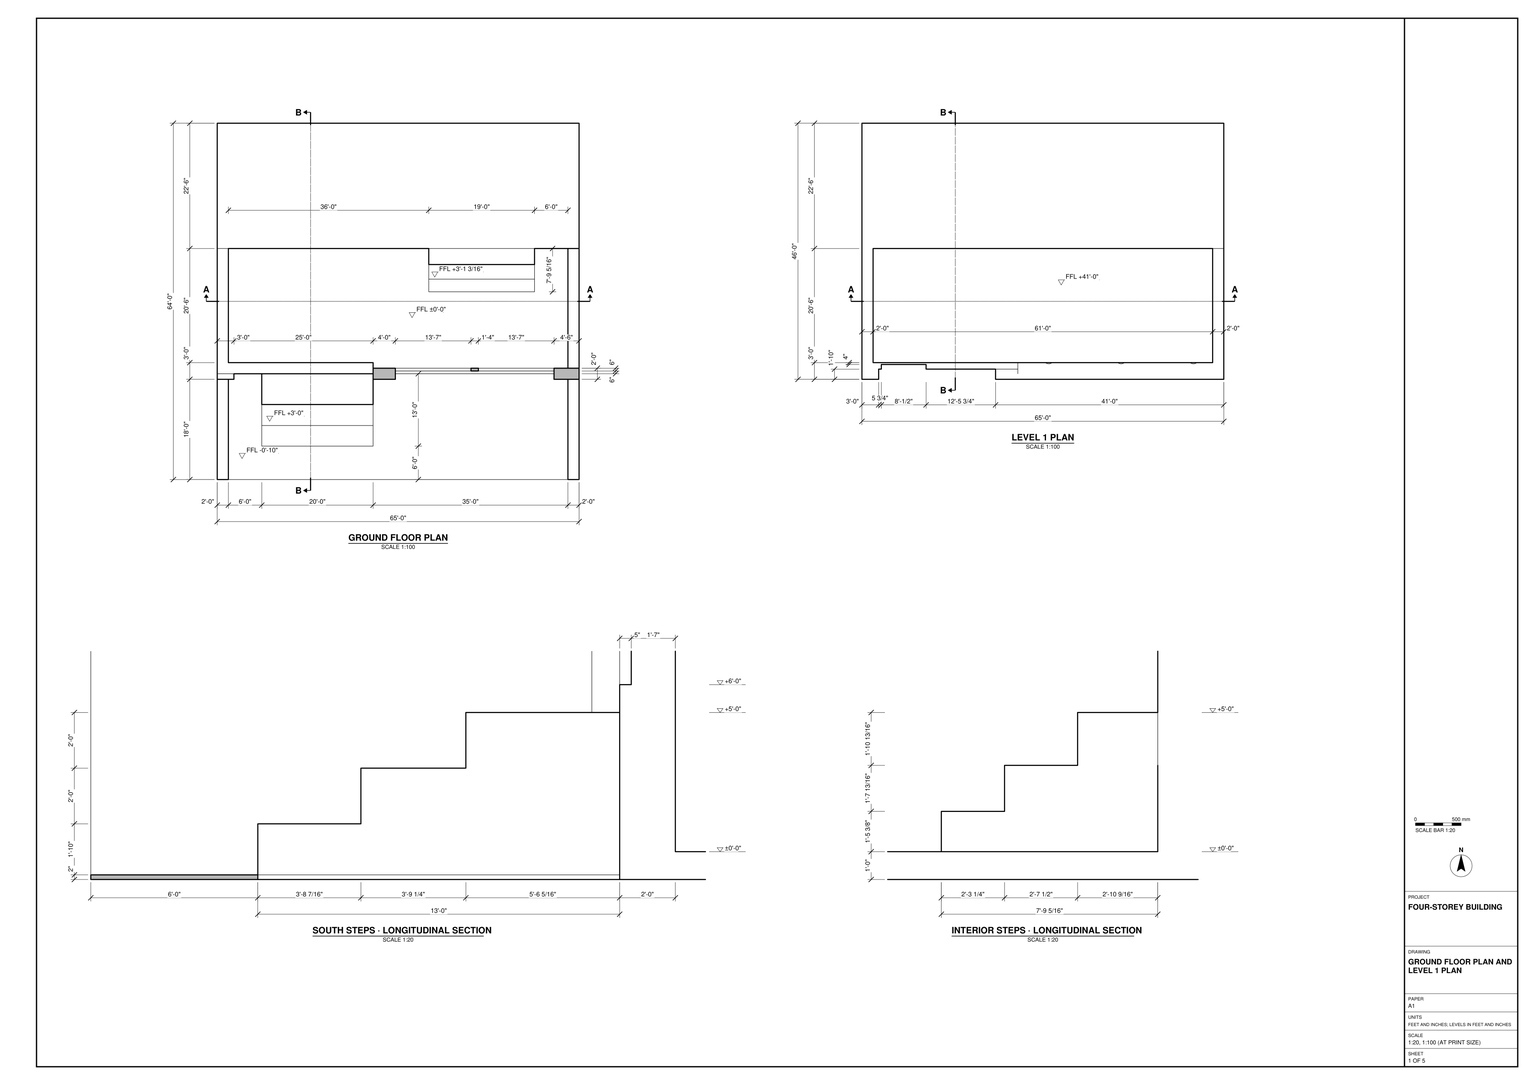
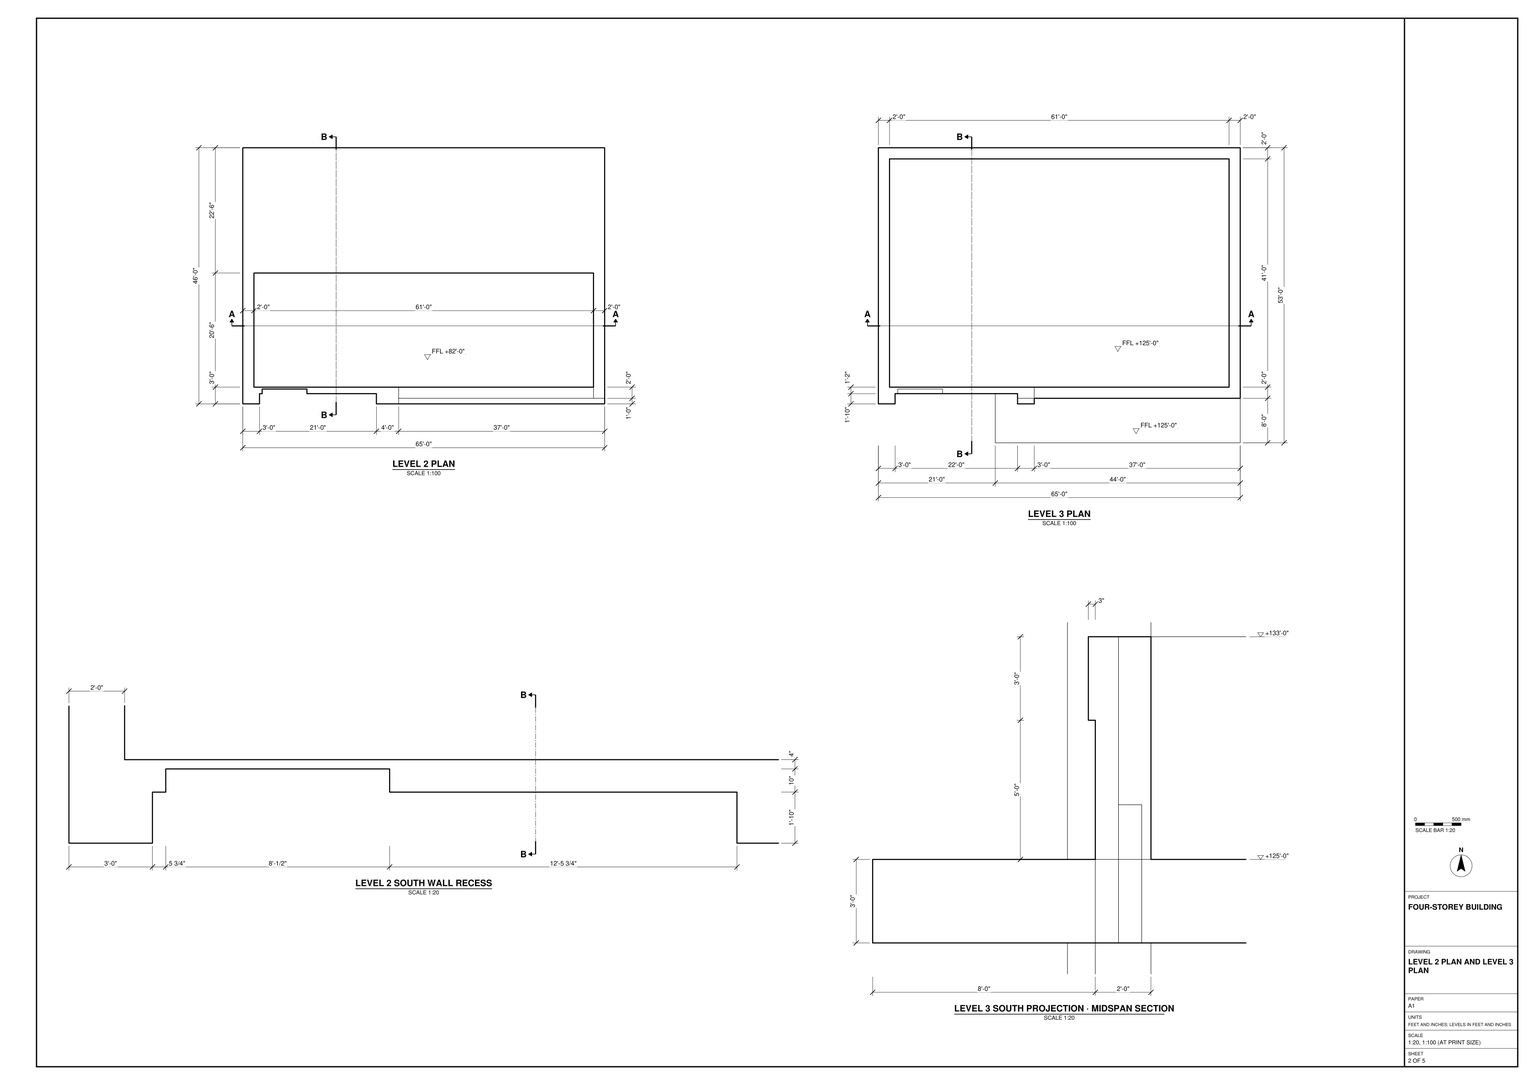
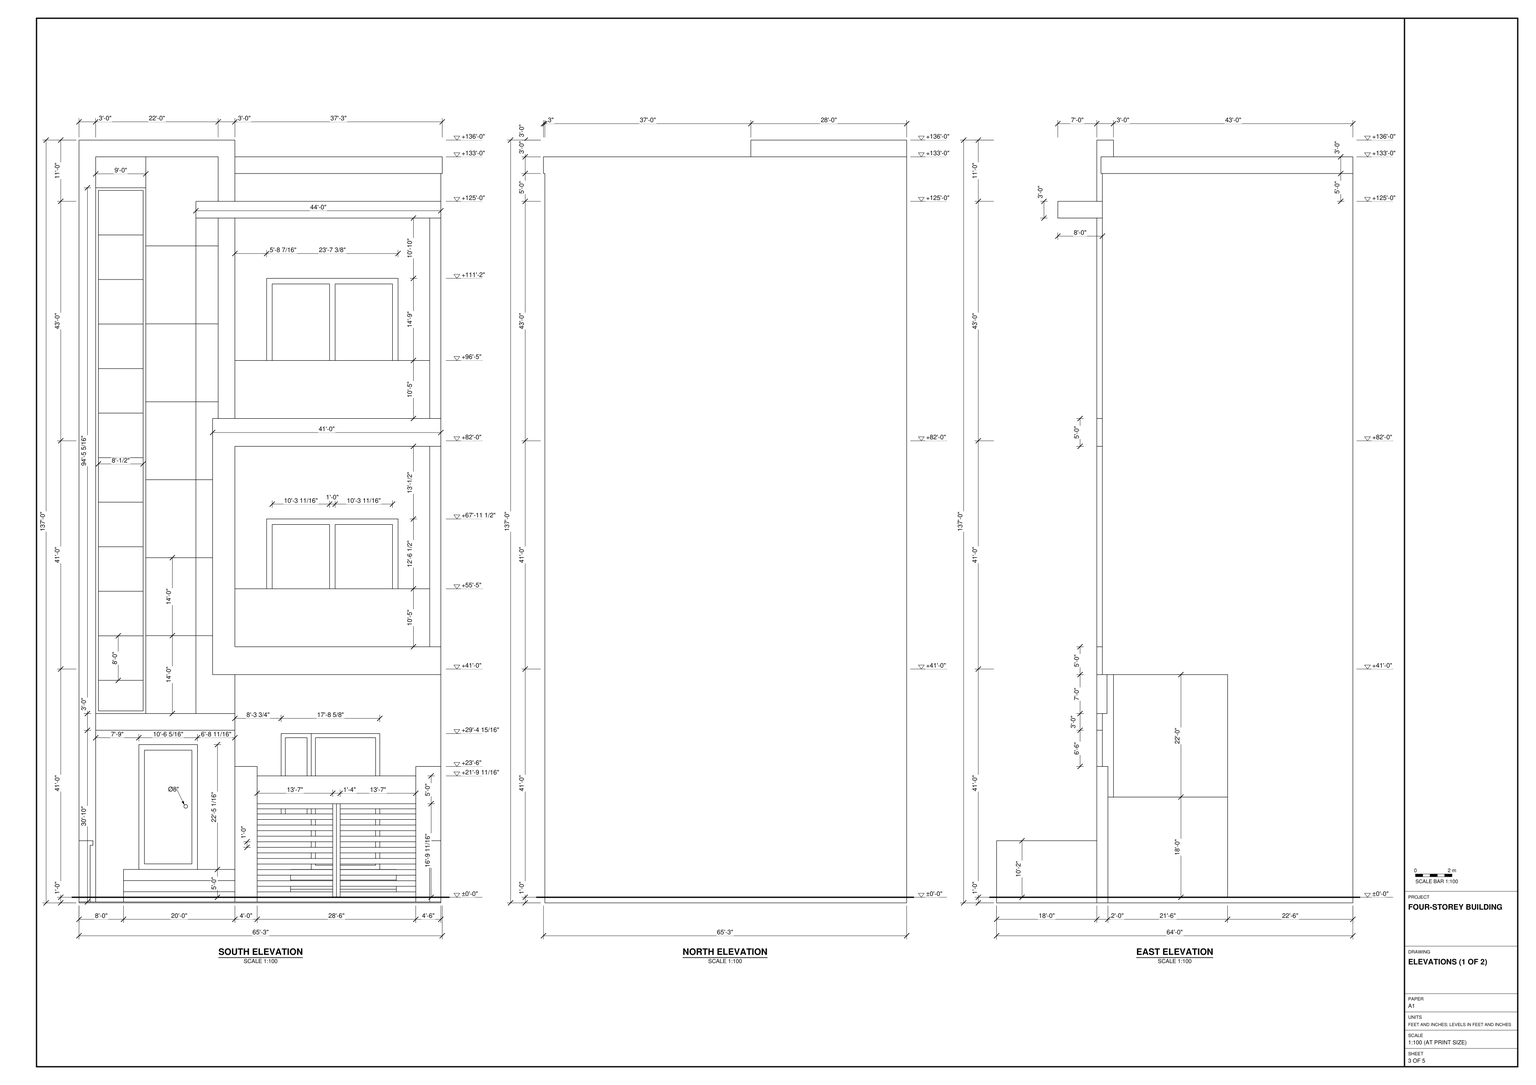
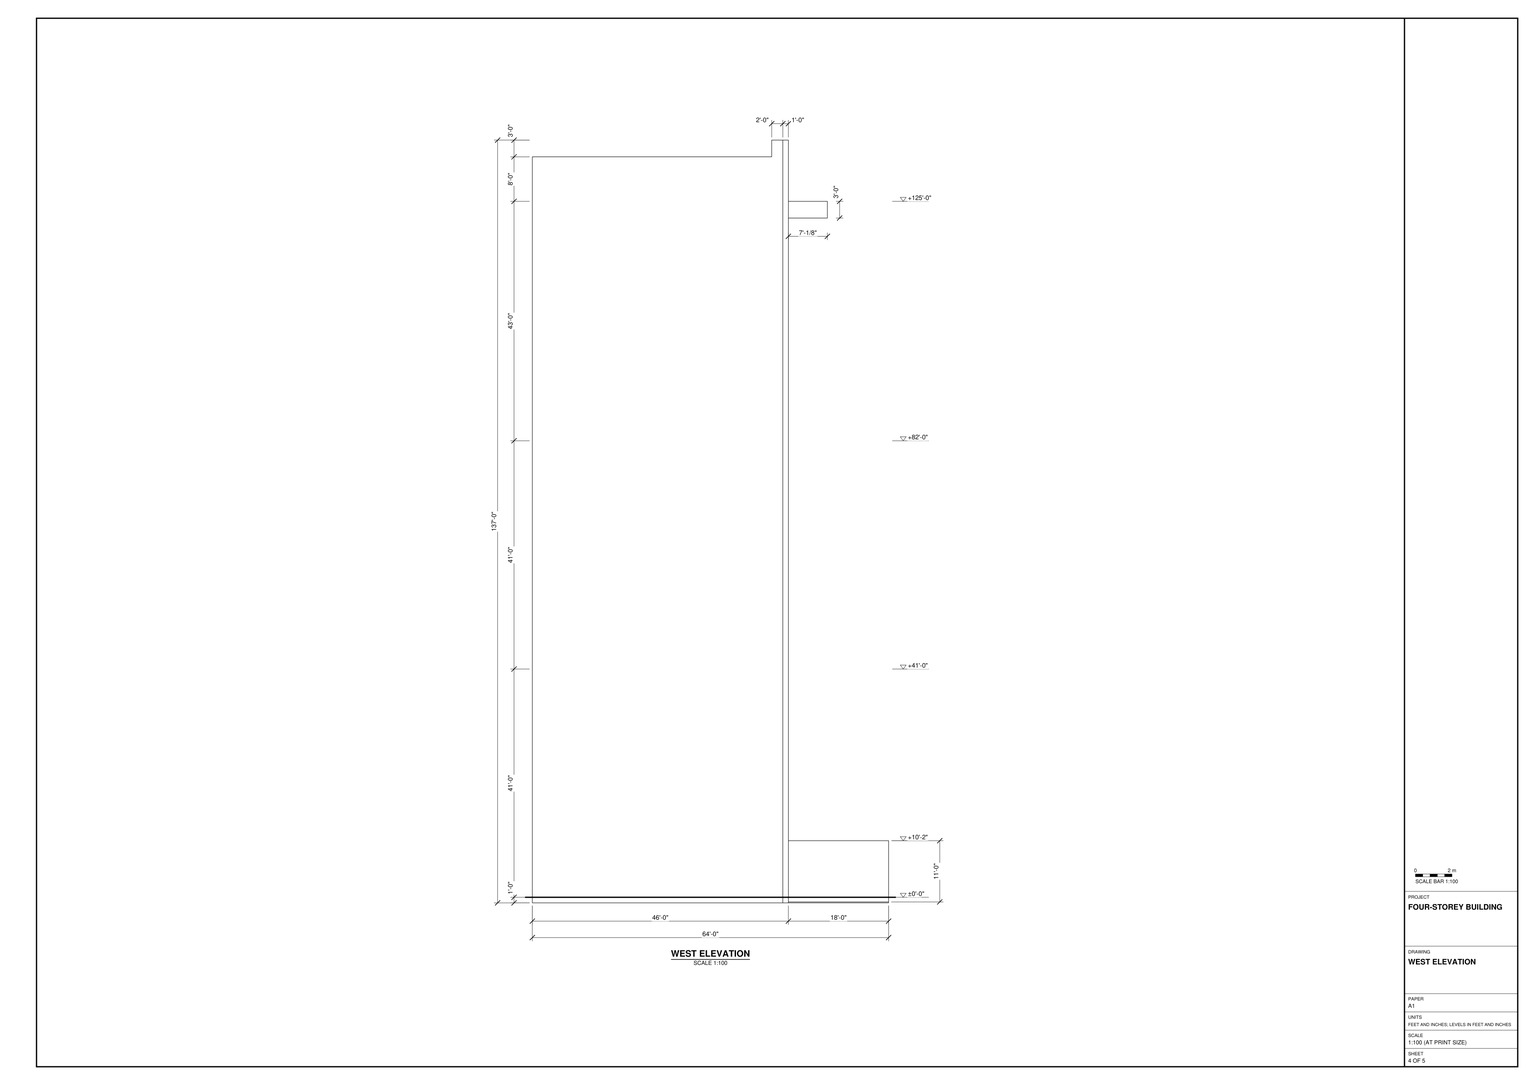
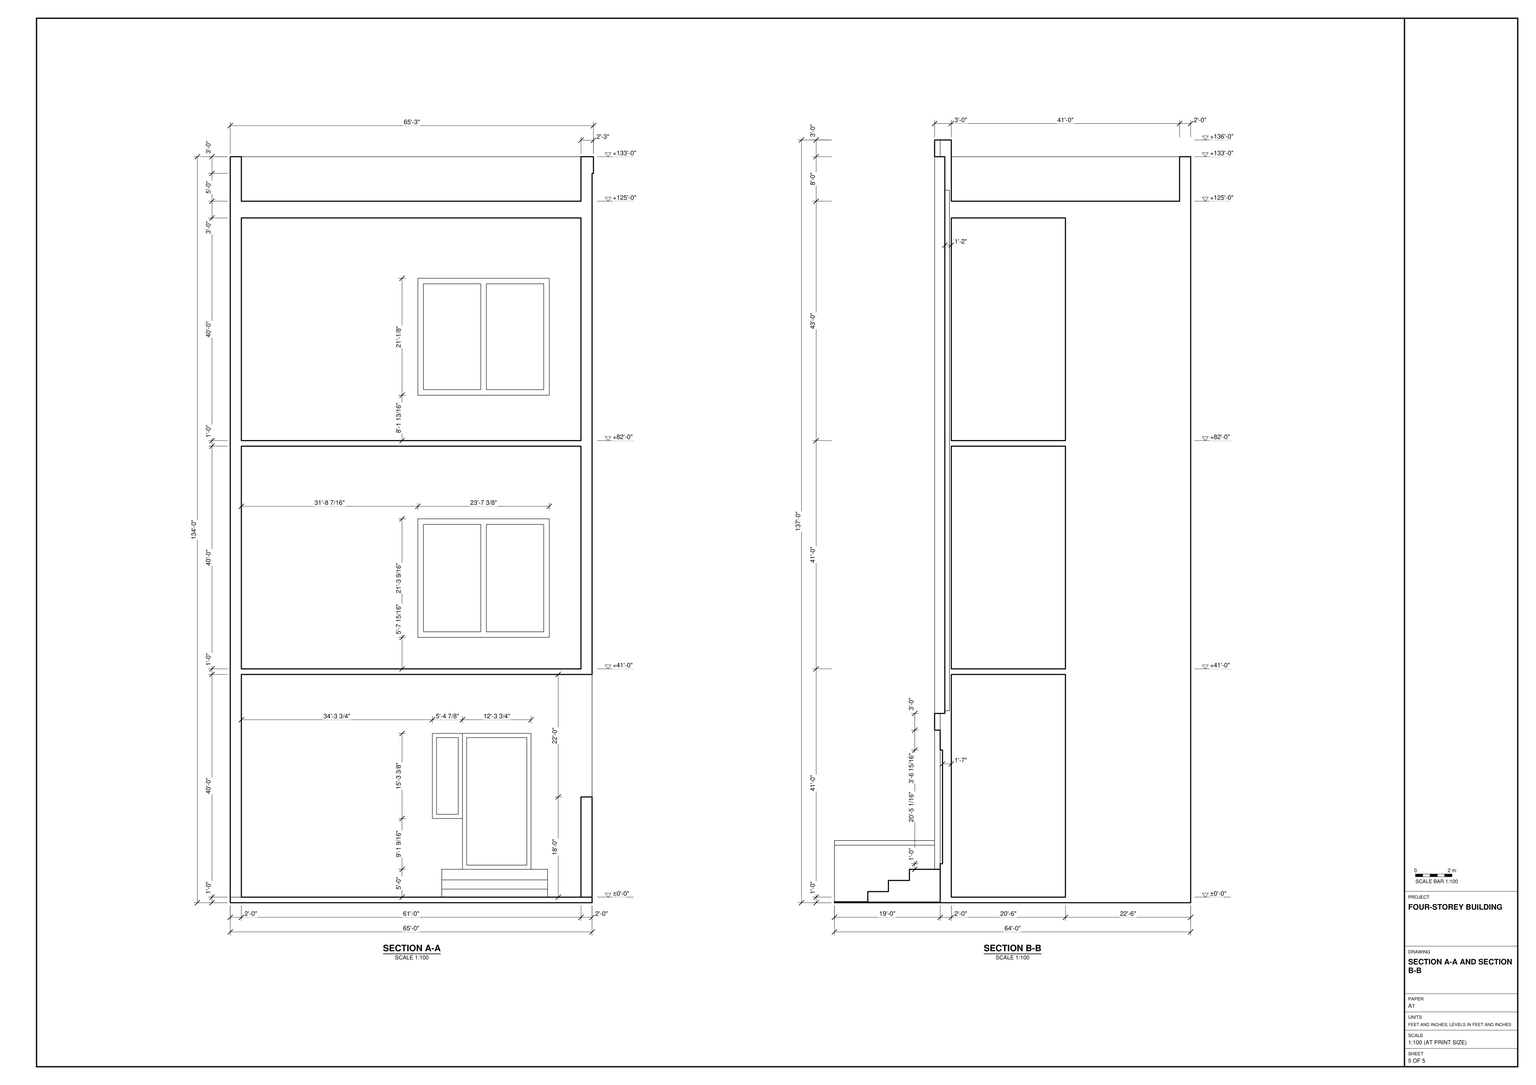
Build the four-storey building in SketchUp from task_files/diagram_01.pdf. Work in feet and inches. Set out the model with an overall east–west width of 65'-3", a north–south depth of 64'-0" and a total height of 137'-0". Use finished floor levels of ±0'-0", +41'-0", +82'-0" and +125'-0".

Follow the plans for the wall thicknesses, slab outlines and setbacks at each level. At ground level, extend the side walls along the south forecourt. Model the broad steps up to the entrance and the separate interior steps using their respective longitudinal sections. Place the entrance door to the left of the horizontal-slat gate as seen in the south elevation.

Build the tall, narrow panelled bay above the entrance and the paired upper-floor openings to its right. Give the facade its drawn depth: form the projecting surrounds, the level 2 wall recess and the level 3 slab projection rather than drawing their outlines on a flat wall. Finish the roof with the stepped parapet profile shown in elevation.

Keep walls, slabs and roof elements in separate groups or components, do the same for each furniture or joinery piece shown, and use components for repeated parts. Any decor or loose items shown may be suitable library components. Save one SketchUp model as output_files/four_storey_building_with_its_stepped_south_facade.skp.

# SketchUp Ruby script. Lengths in inches.
U = 1.inch
M = Sketchup.active_model
def pt(a) = Geom::Point3d.new(a.map { |v| v * U })
def face(e, loops, mat)
  f = e.add_face(loops[0].map { |a| pt(a) })
  loops[1..].each { |l| e.add_face(l.map { |a| pt(a) }).erase! }
  f.material = f.back_material = mat if mat
  f
end
# faces: each face lists its corners as indices into pts; further lists are holes
def faces(e, pts, list, mat = nil) = list.each { |f| face(e, (f[0].is_a?(Array) ? f : [f]).map { |l| l.map { |i| pts[i] } }, mat) }
# xy, xz, yz: faces in a plane at the given z, y or x. An outline is a flat list of corners, or four numbers for a rectangle; further outlines are holes
def ring(l) = l.size == 4 ? [[l[0], l[1]], [l[2], l[1]], [l[2], l[3]], [l[0], l[3]]] : l.each_slice(2).to_a
def flat(e, list, mat, &to3) = list.each { |f| face(e, (f[0].is_a?(Array) ? f : [f]).map { |l| ring(l).map { |u, v| to3.(u, v) } }, mat) }
def xy(e, z, list, mat = nil) = flat(e, list, mat) { |x, y| [x, y, z] }
def xz(e, y, list, mat = nil) = flat(e, list, mat) { |x, z| [x, y, z] }
def yz(e, x, list, mat = nil) = flat(e, list, mat) { |y, z| [x, y, z] }
def lines(e, pts, list) = list.each { |a, b| e.add_line(pt(pts[a]), pt(pts[b])) }
# prism: a flat outline (further loops are holes) pulled along v
def prism(e, loops, v, mat = nil)
  f = face(e, loops, mat); d = Geom::Vector3d.new(v.map { |x| x * U })
  f.pushpull(f.normal.samedirection?(d) ? d.length : -d.length)
end
def box(e, o, s, mat = nil) = prism(e, [[o, [o[0] + s[0], o[1], o[2]], [o[0] + s[0], o[1] + s[1], o[2]], [o[0], o[1] + s[1], o[2]]]], [0, 0, s[2]], mat)
def at(x, y, z, deg = 0) = Geom::Transformation.translation(pt([x, y, z])) * Geom::Transformation.rotation(ORIGIN, Z_AXIS, deg.degrees)
def axes(o, x, y, z) = Geom::Transformation.new([*x, 0, *y, 0, *z, 0, *pt(o).to_a, 1])
def part(name) = M.definitions.add(name)
# library, detail: a bought-in or finely detailed component or shape, given as its bounding box
def library(name, o, s) = part(name).tap { |d| box(d.entities, o, s) }
def detail(e, o, s) = box(e.add_group.entities, o, s)
def put(e, d, t, mat = nil) = e.add_instance(d, t).tap { |i| i.material = mat if mat }
def group(e, t, mat = nil) = e.add_group.tap { |g| g.transformation = t; g.material = mat if mat }.entities
root = M.entities
M.materials.add("[0035_Tan]").color = [178, 153, 119]
M.materials.add("[0111_SlateGray]").color = [41, 47, 53]
M.materials.add("[0135_DarkGray]").color = [81, 81, 81]
M.materials.add("[0137_Black]").color = [0, 0, 0]
M.materials.add("[Cladding Stucco White]").color = [173, 173, 173]
M.materials.add("[Granite Dark Gray]").color = [79, 77, 77]
M.materials.add("[Grass Dark Green]").color = [106, 157, 55]
M.materials.add("[Pavers Driveway Brick]").color = [176, 130, 106]
M.materials.add("[Pavers Flagstone Gray]").color = [162, 162, 162]
M.materials.add("[Stone Masonry Multi]").color = [226, 218, 204]
M.materials.add("[Stone Vein Gray]").color = [166, 165, 165]
M.materials.add("[Translucent Glass Blue]").color = [45, 67, 107]
M.materials["[Translucent Glass Blue]"].alpha = 0.5
M.materials.add("[Translucent Glass Gray]").color = [211, 211, 211]
M.materials["[Translucent Glass Gray]"].alpha = 0.5
M.materials.add("[Translucent Glass Gray]1").color = [128, 128, 128]
M.materials["[Translucent Glass Gray]1"].alpha = 0.5
M.materials.add("[Wood Bamboo]").color = [177, 105, 43]
M.materials.add("[Wood Veneer 01]").color = [120, 70, 37]
xy(root,0,[[0,0,0,216,36,216,36,228,96,228,96,72,336,72,336,216,384,216,384,228,726,228,726,216,780,216,780,0],[96,72,336,228],[0,216,36,228],[336,216,384,228],[726,216,780,228],
  [0,228,780,768]])
xy(root,2,[[0,0,24,216]])
xy(root,2,[[24,0,756,0,756,216,726,216,726,228,384,228,384,216,336,216,336,72,96,72,96,228,36,228,36,216,24,216]],"[Pavers Driveway Brick]")
xy(root,12,[[384,234,726,240],[756,240,780,498],[456,404.6875,684,498]])
xy(root,12,[[384,228,726,234],[336,240,756,240,756,498,684,498,684,404.6875,456,404.6875,456,498,24,498,24,252,336,252]],"[Granite Dark Gray]")
xy(root,23.6875,[[384,234,547,240],[563,234,726,240]],"[0135_DarkGray]")
xy(root,24,[[96,72,336,116.4375]],"[Cladding Stucco White]")
xy(root,29.36,[[456,404.6875,684,431.9375]],"[Stone Vein Gray]")
xy(root,35.6875,[[384,234,547,240],[563,234,726,240]])
xy(root,47.6875,[[384,234,547,240],[563,234,726,240]],"[0135_DarkGray]")
xy(root,48,[[96,116.4375,336,161.6875]],"[Cladding Stucco White]")
xy(root,49.2,[[456,431.9375,684,463.4375]],"[Stone Vein Gray]")
xy(root,59.6875,[[384,234,547,240],[563,234,726,240]])
xy(root,71.6875,[[384,234,547,240],[563,234,726,240]],"[0135_DarkGray]")
xy(root,72,[[96,161.6875,336,228]],"[Cladding Stucco White]")
xy(root,72,[[456,463.4375,684,498]],"[Stone Vein Gray]")
xy(root,83.6875,[[384,234,547,240],[563,234,726,240]])
xy(root,84,[[141.01,228,243.33,233]],"[Wood Bamboo]")
xy(root,95.6875,[[384,234,547,240],[563,234,726,240]],"[0135_DarkGray]")
xy(root,107.6875,[[384,234,547,240],[563,234,726,240]])
xy(root,119.6875,[[384,234,547,240],[563,234,726,240]],"[0135_DarkGray]")
xy(root,124,[[24,0,30,216],[750,0,756,216]],"[0135_DarkGray]")
xy(root,131.6875,[[384,234,547,240],[563,234,726,240]])
xy(root,134,[[0,0,30,216],[750,0,780,216]],"[0135_DarkGray]")
xy(root,143.6875,[[384,234,547,240],[563,234,726,240]],"[0135_DarkGray]")
xy(root,155.6875,[[384,234,547,240],[563,234,726,240]])
xy(root,167.6875,[[384,234,547,240],[563,234,726,240]],"[0135_DarkGray]")
xy(root,179.6875,[[384,234,547,240],[563,234,726,240]])
xy(root,191.6875,[[384,234,547,240],[563,234,726,240]],"[0135_DarkGray]")
xy(root,202.6875,[[384,234,547,240],[563,234,726,240]])
xy(root,228,[[756,240,780,498]])
xy(root,273.6875,[[384,234,726,240]],"[0135_DarkGray]")
xy(root,294,[[336,216,384,240],[726,216,780,240]],"[0111_SlateGray]")
xy(root,329.0625,[[141.01,228,243.33,233]],"[Wood Bamboo]")
xy(root,372,[[36,216,336,228]])
xy(root,408,[[36,216,336,238]],"[0135_DarkGray]")
xy(root,413.74,[[41.74,238,138.26,248]],"[0135_DarkGray]")
xy(root,492,[[402.42,249.38,399.58,249.81,396.95,250.95,394.7,252.74,392.99,255.05,391.9375,257.72,391.61,260.57,392.04,263.41,393.18,266.05,394.97,268.29,397.28,270,399.95,271.05,402.8,271.38,405.64,270.95,408.28,269.81,410.52,268.02,412.23,265.71,413.28,263.04,413.61,260.1875,413.18,257.35,412.04,254.72,410.25,252.47,407.94,250.76,405.27,249.71],[558.42,249.38,555.58,249.81,552.95,250.95,550.7,252.74,548.99,255.05,547.9375,257.72,547.61,260.57,548.04,263.41,549.18,266.05,550.97,268.29,553.28,270,555.95,271.05,558.8,271.38,561.64,270.95,564.28,269.81,566.52,268.02,568.23,265.71,569.28,263.04,569.61,260.1875,569.18,257.35,568.04,254.72,566.25,252.47,563.94,250.76,561.27,249.71],[714.42,249.38,711.58,249.81,708.95,250.95,706.7,252.74,704.99,255.05,703.9375,257.72,703.61,260.57,704.04,263.41,705.18,266.05,706.97,268.29,709.28,270,711.95,271.05,714.8,271.38,717.64,270.95,720.28,269.81,722.52,268.02,724.23,265.71,725.28,263.04,725.61,260.1875,725.18,257.35,724.04,254.72,722.25,252.47,719.94,250.76,717.27,249.71]])
xy(root,492,[[[288,216,288,238,336,238,336,252,24,252,24,498,780,498,780,216],[402.42,249.38,405.27,249.71,407.94,250.76,410.25,252.47,412.04,254.72,413.18,257.35,413.61,260.1875,413.28,263.04,412.23,265.71,410.52,268.02,408.28,269.81,405.64,270.95,402.8,271.38,399.95,271.05,397.28,270,394.97,268.29,393.18,266.05,392.04,263.41,391.61,260.57,391.9375,257.72,392.99,255.05,394.7,252.74,396.95,250.95,399.58,249.81],[558.42,249.38,561.27,249.71,563.94,250.76,566.25,252.47,568.04,254.72,569.18,257.35,569.61,260.1875,569.28,263.04,568.23,265.71,566.52,268.02,564.28,269.81,561.64,270.95,558.8,271.38,555.95,271.05,553.28,270,550.97,268.29,549.18,266.05,548.04,263.41,547.61,260.57,547.9375,257.72,548.99,255.05,550.7,252.74,552.95,250.95,555.58,249.81],[714.42,249.38,717.27,249.71,719.94,250.76,722.25,252.47,724.04,254.72,725.18,257.35,725.61,260.1875,725.28,263.04,724.23,265.71,722.52,268.02,720.28,269.81,717.64,270.95,714.8,271.38,711.95,271.05,709.28,270,706.97,268.29,705.18,266.05,704.04,263.41,703.61,260.57,703.9375,257.72,704.99,255.05,706.7,252.74,708.95,250.95,711.58,249.81]]],"[Wood Veneer 01]")
xy(root,504,[[24,252,756,498]],"[Grass Dark Green]")
xy(root,552,[[336,240,756,252]])
xy(root,552,[[336,216,780,216,780,228,756,228,756,240,336,240]],"[0135_DarkGray]")
xy(root,984,[[336,216,780,228],[349.97,358.37,347.36,358.41,344.85,359.13,342.62,360.48,340.8,362.36,339.54,364.64,338.91,367.18,338.96,369.79,339.68,372.3,341.02,374.53,342.9,376.34,345.1875,377.61,347.72,378.24,350.33,378.19,352.84,377.47,355.08,376.125,356.89,374.24,358.15,371.96,358.78,369.43,358.73,366.82,358.01,364.31,356.67,362.07,354.79,360.26,352.5,359],[517.97,358.37,515.36,358.41,512.85,359.13,510.62,360.48,508.8,362.36,507.54,364.64,506.91,367.18,506.96,369.79,507.68,372.3,509.02,374.53,510.9,376.34,513.1875,377.61,515.72,378.24,518.33,378.19,520.84,377.47,523.08,376.125,524.89,374.24,526.15,371.96,526.78,369.43,526.73,366.82,526.01,364.31,524.67,362.07,522.79,360.26,520.5,359],[685.97,358.37,683.36,358.41,680.85,359.13,678.62,360.48,676.8,362.36,675.54,364.64,674.91,367.18,674.96,369.79,675.68,372.3,677.02,374.53,678.9,376.34,681.1875,377.61,683.72,378.24,686.33,378.19,688.84,377.47,691.08,376.125,692.89,374.24,694.15,371.96,694.78,369.43,694.73,366.82,694.01,364.31,692.67,362.07,690.79,360.26,688.5,359]])
xy(root,984,[[[336,228,336,252,24,252,24,498,756,498,756,228],[349.97,358.37,352.5,359,354.79,360.26,356.67,362.07,358.01,364.31,358.73,366.82,358.78,369.43,358.15,371.96,356.89,374.24,355.08,376.125,352.84,377.47,350.33,378.19,347.72,378.24,345.1875,377.61,342.9,376.34,341.02,374.53,339.68,372.3,338.96,369.79,338.91,367.18,339.54,364.64,340.8,362.36,342.62,360.48,344.85,359.13,347.36,358.41],[517.97,358.37,520.5,359,522.79,360.26,524.67,362.07,526.01,364.31,526.73,366.82,526.78,369.43,526.15,371.96,524.89,374.24,523.08,376.125,520.84,377.47,518.33,378.19,515.72,378.24,513.1875,377.61,510.9,376.34,509.02,374.53,507.68,372.3,506.96,369.79,506.91,367.18,507.54,364.64,508.8,362.36,510.62,360.48,512.85,359.13,515.36,358.41],[685.97,358.37,688.5,359,690.79,360.26,692.67,362.07,694.01,364.31,694.73,366.82,694.78,369.43,694.15,371.96,692.89,374.24,691.08,376.125,688.84,377.47,686.33,378.19,683.72,378.24,681.1875,377.61,678.9,376.34,677.02,374.53,675.68,372.3,674.96,369.79,674.91,367.18,675.54,364.64,676.8,362.36,678.62,360.48,680.85,359.13,683.36,358.41]]],"[Wood Veneer 01]")
xy(root,996,[[24,252,756,498]],"[Grass Dark Green]")
xy(root,1044,[[336,240,756,252]])
xy(root,1044,[[288,216,780,216,780,228,756,228,756,240,336,240,336,228,300,228,300,238,288,238]],"[0135_DarkGray]")
xy(root,1476,[[397.37,251.66,392.79,252.7,388.63,254.89,385.18,258.08,382.67,262.06,381.28,266.54,381.09,271.24,382.13,275.82,384.32,279.98,387.51,283.43,391.49,285.9375,395.97,287.33,400.67,287.51,405.25,286.47,409.41,284.29,412.86,281.1,415.37,277.12,416.76,272.63,416.94,267.9375,415.91,263.36,413.72,259.2,410.53,255.75,406.55,253.24,402.0625,251.85],[529.37,251.66,524.79,252.7,520.63,254.89,517.18,258.08,514.67,262.06,513.28,266.54,513.09,271.24,514.13,275.82,516.32,279.98,519.51,283.43,523.49,285.9375,527.97,287.33,532.67,287.51,537.25,286.47,541.41,284.29,544.86,281.1,547.37,277.12,548.76,272.63,548.94,267.9375,547.91,263.36,545.72,259.2,542.53,255.75,538.55,253.24,534.0625,251.85],[661.37,251.66,656.79,252.7,652.63,254.89,649.18,258.08,646.67,262.06,645.28,266.54,645.09,271.24,646.13,275.82,648.32,279.98,651.51,283.43,655.49,285.9375,659.97,287.33,664.67,287.51,669.25,286.47,673.41,284.29,676.86,281.1,679.37,277.12,680.76,272.63,680.94,267.9375,679.91,263.36,677.72,259.2,674.53,255.75,670.55,253.24,666.0625,251.85],[399.93,383.66,395.35,384.7,391.19,386.89,387.74,390.08,385.23,394.06,383.84,398.54,383.66,403.24,384.7,407.82,386.88,411.98,390.07,415.43,394.05,417.9375,398.54,419.33,403.23,419.51,407.81,418.47,411.97,416.29,415.42,413.1,417.93,409.12,419.32,404.63,419.51,399.9375,418.47,395.36,416.28,391.2,413.09,387.75,409.11,385.24,404.625,383.85],[529.37,383.66,524.79,384.7,520.63,386.89,517.18,390.08,514.67,394.06,513.28,398.54,513.09,403.24,514.13,407.82,516.32,411.98,519.51,415.43,523.49,417.9375,527.97,419.33,532.67,419.51,537.25,418.47,541.41,416.29,544.86,413.1,547.37,409.12,548.76,404.63,548.94,399.9375,547.91,395.36,545.72,391.2,542.53,387.75,538.55,385.24,534.0625,383.85],
  [661.37,383.66,656.79,384.7,652.63,386.89,649.18,390.08,646.67,394.06,645.28,398.54,645.09,403.24,646.13,407.82,648.32,411.98,651.51,415.43,655.49,417.9375,659.97,419.33,664.67,419.51,669.25,418.47,673.41,416.29,676.86,413.1,679.37,409.12,680.76,404.63,680.94,399.9375,679.91,395.36,677.72,391.2,674.53,387.75,670.55,385.24,666.0625,383.85]])
xy(root,1476,[[[252,132,252,238,300,238,300,228,336,228,336,252,24,252,24,498,756,498,756,228,780,228,780,132],[397.37,251.66,402.0625,251.85,406.55,253.24,410.53,255.75,413.72,259.2,415.91,263.36,416.94,267.9375,416.76,272.63,415.37,277.12,412.86,281.1,409.41,284.29,405.25,286.47,400.67,287.51,395.97,287.33,391.49,285.9375,387.51,283.43,384.32,279.98,382.13,275.82,381.09,271.24,381.28,266.54,382.67,262.06,385.18,258.08,388.63,254.89,392.79,252.7],[529.37,251.66,534.0625,251.85,538.55,253.24,542.53,255.75,545.72,259.2,547.91,263.36,548.94,267.9375,548.76,272.63,547.37,277.12,544.86,281.1,541.41,284.29,537.25,286.47,532.67,287.51,527.97,287.33,523.49,285.9375,519.51,283.43,516.32,279.98,514.13,275.82,513.09,271.24,513.28,266.54,514.67,262.06,517.18,258.08,520.63,254.89,524.79,252.7],[661.37,251.66,666.0625,251.85,670.55,253.24,674.53,255.75,677.72,259.2,679.91,263.36,680.94,267.9375,680.76,272.63,679.37,277.12,676.86,281.1,673.41,284.29,669.25,286.47,664.67,287.51,659.97,287.33,655.49,285.9375,651.51,283.43,648.32,279.98,646.13,275.82,645.09,271.24,645.28,266.54,646.67,262.06,649.18,258.08,652.63,254.89,656.79,252.7],[529.37,383.66,534.0625,383.85,538.55,385.24,542.53,387.75,545.72,391.2,547.91,395.36,548.94,399.9375,548.76,404.63,547.37,409.12,544.86,413.1,541.41,416.29,537.25,418.47,532.67,419.51,527.97,419.33,523.49,417.9375,519.51,415.43,516.32,411.98,514.13,407.82,513.09,403.24,513.28,398.54,514.67,394.06,517.18,390.08,520.63,386.89,524.79,384.7],[399.93,383.66,404.625,383.85,409.11,385.24,413.09,387.75,416.28,391.2,418.47,395.36,419.51,399.9375,419.32,404.63,417.93,409.12,415.42,413.1,411.97,416.29,407.81,418.47,403.23,419.51,398.54,419.33,394.05,417.9375,390.07,415.43,386.88,411.98,384.7,407.82,383.66,403.24,383.84,398.54,385.23,394.06,387.74,390.08,391.19,386.89,395.35,384.7],[661.37,383.66,666.0625,383.85,670.55,385.24,674.53,387.75,677.72,391.2,679.91,395.36,680.94,399.9375,680.76,404.63,679.37,409.12,676.86,413.1,673.41,416.29,669.25,418.47,664.67,419.51,659.97,419.33,655.49,417.9375,651.51,415.43,648.32,411.98,646.13,407.82,645.09,403.24,645.28,398.54,646.67,394.06,649.18,390.08,652.63,386.89,656.79,384.7]]],"[Wood Veneer 01]")
xy(root,1512,[[300,216,336,228],[24,252,756,744]])
xy(root,1512,[[252,132,780,132,780,228,336,228,336,216,300,216,300,238,252,238]],"[0135_DarkGray]")
xy(root,1535.57,[[41.74,238,138.26,248]],"[0135_DarkGray]")
xy(root,1572,[[336,225,336,228,780,228,780,768,783,768,783,225]])
xy(root,1608,[[36,216,300,238],[336,225,783,225,783,768,0,768,0,252,24,252,24,744,756,744,756,252,336,252]])
xy(root,1644,[[0,216,336,252]])
xz(root,0,[[0,0,780,2]])
xz(root,0,[[0,2,24,2,24,124,30,124,30,134,0,134],[756,2,780,2,780,134,750,134,750,124,756,124]],"[Cladding Stucco White]")
xz(root,72,[[96,0,336,2]])
xz(root,72,[[96,2,336,24]],"[Cladding Stucco White]")
xz(root,116.4375,[[96,24,336,48]],"[Cladding Stucco White]")
xz(root,132,[[252,1476,780,1512]],"[0135_DarkGray]")
xz(root,161.6875,[[96,48,336,72]],"[Cladding Stucco White]")
xz(root,216,[[0,0,36,2],[336,0,384,2],[726,0,780,2],[0,2,24,134],[756,2,780,134],
  [24,124,30,134],[750,124,756,134]])
xz(root,216,[[336,2,384,294],[726,2,756,2,756,124,750,124,750,134,780,134,780,294,726,294]],"[0111_SlateGray]")
xz(root,216,[[24,2,36,2,36,1608,300,1608,300,1512,336,1512,336,1644,0,1644,0,134,30,134,30,124,24,124],[36,372,336,408],[288,492,780,492,780,552,336,552,336,984,780,984,780,1044,288,1044]],"[0135_DarkGray]")
xz(root,225,[[336,1572,783,1608]],"[0135_DarkGray]")
xz(root,228,[[36,0,96,2],[96,0,336,24],[384,0,726,2],[36,2,96,2,96,72,129.01,72,129.01,341.0625,255.33,341.0625,255.33,72,336,72,336,372,36,372],[96,24,336,48],
  [96,48,336,72],[336,1512,780,1572]])
xz(root,228,[[756,552,780,984],[300,1044,336,1476],[756,1044,780,1476]],"[0135_DarkGray]")
xz(root,228,[[384,2,726,12]],"[Granite Dark Gray]")
xz(root,228,[[[129.01,72,255.33,341.0625],[141.01,84,243.33,329.0625]]],"[Wood Bamboo]")
xz(root,233,[[230.0625,204.02,231.1,204.16,232.0625,204.56,232.89,205.19,233.53,206.02,233.93,206.99,234.0625,208.02,233.93,209.06,233.53,210.02,232.89,210.85,232.0625,211.49,231.1,211.88,230.0625,212.02,229.03,211.88,228.0625,211.49,227.23,210.85,226.6,210.02,226.2,209.06,226.0625,208.02,226.2,206.99,226.6,206.02,227.23,205.19,228.0625,204.56,229.03,204.16]])
xz(root,233,[[[141.01,84,243.33,329.0625],[230.0625,204.02,229.03,204.16,228.0625,204.56,227.23,205.19,226.6,206.02,226.2,206.99,226.0625,208.02,226.2,209.06,226.6,210.02,227.23,210.85,228.0625,211.49,229.03,211.88,230.0625,212.02,231.1,211.88,232.0625,211.49,232.89,210.85,233.53,210.02,233.93,209.06,234.0625,208.02,233.93,206.99,233.53,206.02,232.89,205.19,232.0625,204.56,231.1,204.16]]],"[Wood Bamboo]")
xz(root,234,[[384,12,547,23.6875],[547,12,555,213.6875],[555,12,563,213.6875],[563,12,726,23.6875],[384,35.6875,547,47.6875],
  [563,35.6875,726,47.6875],[384,59.6875,547,71.6875],[563,59.6875,726,71.6875],[384,83.6875,547,95.6875],[563,83.6875,726,95.6875],
  [384,107.6875,547,119.6875],[563,107.6875,726,119.6875],[384,131.6875,547,143.6875],[563,131.6875,726,143.6875],[384,155.6875,547,167.6875],
  [563,155.6875,726,167.6875],[384,179.6875,547,191.6875],[563,179.6875,726,191.6875],[384,202.6875,547,213.6875],[563,202.6875,726,213.6875],
  [384,213.6875,726,273.6875]],"[0135_DarkGray]")
xz(root,238,[[[36,408,144,1541.32],[41.74,413.74,138.26,1535.57]],[36,1541.32,144,1608]],"[0135_DarkGray]")
xz(root,238,[[144,408,252,576],[252,408,336,408,336,492,288,492,288,576,252,576],[144,576,252,744],[252,576,288,744],[144,744,252,912],
  [252,744,288,912],[144,912,252,1080],[252,912,288,912,288,1044,300,1044,300,1080,252,1080],[144,1080,252,1248],[252,1080,300,1248],
  [144,1248,252,1416],[252,1248,300,1416],[144,1416,252,1416,252,1512,300,1512,300,1608,144,1608],[252,1416,300,1476]],"[Pavers Flagstone Gray]")
xz(root,240,[[756,12,780,228],[336,667,756,672],[336,1159,756,1164]])
xz(root,240,[[336,12,384,294],[726,12,726,294,780,294,780,228,756,228,756,12]],"[0111_SlateGray]")
xz(root,240,[[384,12,384,23.6875,547,23.6875,547,35.6875,384,35.6875,384,47.6875,547,47.6875,547,59.6875,384,59.6875,384,71.6875,547,71.6875,547,83.6875,384,83.6875,384,95.6875,547,95.6875,547,107.6875,384,107.6875,384,119.6875,547,119.6875,547,131.6875,384,131.6875,384,143.6875,547,143.6875,547,155.6875,384,155.6875,384,167.6875,547,167.6875,547,179.6875,384,179.6875,384,191.6875,547,191.6875,547,202.6875,384,202.6875,384,273.6875,726,273.6875,726,202.6875,563,202.6875,563,191.6875,726,191.6875,726,179.6875,563,179.6875,563,167.6875,726,167.6875,726,155.6875,563,155.6875,563,143.6875,726,143.6875,726,131.6875,563,131.6875,563,119.6875,726,119.6875,726,107.6875,563,107.6875,563,95.6875,726,95.6875,726,83.6875,563,83.6875,563,71.6875,726,71.6875,726,59.6875,563,59.6875,563,47.6875,726,47.6875,726,35.6875,563,35.6875,563,23.6875,726,23.6875,726,12]],"[0135_DarkGray]")
xz(root,240,[[336,552,756,667],[336,1044,756,1159]],"[Translucent Glass Gray]1")
xz(root,248,[[41.74,413.74,138.26,479.57],[41.74,479.57,138.26,575.57],[41.74,575.57,138.26,671.57],[41.74,671.57,138.26,767.57],[41.74,767.57,138.26,863.57],
  [41.74,863.57,138.26,959.57],[41.74,959.57,138.26,1055.57],[41.74,1055.57,138.26,1151.57],[41.74,1151.57,138.26,1247.57],[41.74,1247.57,138.26,1343.57],
  [41.74,1343.57,138.26,1439.57],[41.74,1439.57,138.26,1535.57]],"[Translucent Glass Blue]")
xz(root,252,[[336,504,756,552],[336,996,756,1044],[24,1512,24,1608,0,1608,0,1644,336,1644,336,1608,756,1608,756,1512]])
xz(root,252,[[24,12,336,492],[24,996,336,1476]],"[0035_Tan]")
xz(root,252,[[24,504,336,984]],"[Wood Bamboo]")
xz(root,404.6875,[[456,12,684,29.36]],"[Stone Vein Gray]")
xz(root,431.9375,[[456,29.36,684,49.2]],"[Stone Vein Gray]")
xz(root,463.4375,[[456,49.2,684,72]],"[Stone Vein Gray]")
xz(root,498,[[456,12,684,29.36],[756,12,780,228],[456,29.36,684,49.2]])
xz(root,498,[[[500.64,72,648.39,364.9375],[509.64,81,639.39,355.9375]],[[435.76,181.5625,500.64,364.9375],[444.76,190.5625,491.64,355.9375]],[[404.42,571.94,687.8,827.51],[552.11,583.94,675.8,815.51],[416.42,583.94,540.11,815.51]],[[404.42,1093.84,687.8,1345.99],[416.42,1105.84,540.11,1333.99],[552.11,1105.84,675.8,1333.99]]],"[0137_Black]")
xz(root,498,[[24,12,456,12,456,72,500.64,72,500.64,181.5625,435.76,181.5625,435.76,364.9375,648.39,364.9375,648.39,72,684,72,684,12,756,12,756,228,780,228,780,492,24,492],[[24,996,756,1476],[404.42,1093.84,687.8,1345.99]]],"[Stone Masonry Multi]")
xz(root,498,[[509.64,81,639.39,355.9375],[444.76,190.5625,491.64,355.9375],[416.42,583.94,540.11,815.51],[552.11,583.94,675.8,815.51],[416.42,1105.84,540.11,1333.99],
  [552.11,1105.84,675.8,1333.99]],"[Translucent Glass Gray]")
xz(root,498,[[[24,504,756,984],[404.42,571.94,687.8,827.51]]],"[Wood Bamboo]")
xz(root,744,[[24,1512,756,1608]])
xz(root,768,[[0,0,780,12],[0,12,0,1608,783,1608,783,1572,780,1572,780,12]])
yz(root,0,[[0,0,216,2],[216,0,228,1644],[228,0,228,1644,252,1644,252,1608,768,1608,768,0]])
yz(root,0,[[0,2,216,134]],"[Cladding Stucco White]")
yz(root,24,[[252,1512,744,1608]])
yz(root,24,[[252,12,498,492],[252,996,498,1476]],"[0035_Tan]")
yz(root,24,[[0,2,216,124]],"[Cladding Stucco White]")
yz(root,24,[[252,504,498,984]],"[Wood Bamboo]")
yz(root,30,[[0,124,216,134]],"[0135_DarkGray]")
yz(root,36,[[216,0,228,2],[216,372,228,408]])
yz(root,36,[[216,2,228,372],[216,408,238,1608]],"[0135_DarkGray]")
yz(root,41.74,[[238,413.74,248,1535.57]],"[0135_DarkGray]")
yz(root,96,[[72,0,228,2]])
yz(root,96,[[72,2,72,24,116.4375,24,116.4375,48,161.6875,48,161.6875,72,228,72,228,2]],"[Cladding Stucco White]")
yz(root,138.26,[[238,413.74,248,1535.57]],"[0135_DarkGray]")
yz(root,141.01,[[228,84,233,329.0625]],"[Wood Bamboo]")
yz(root,243.33,[[228,84,233,329.0625]],"[Wood Bamboo]")
yz(root,252,[[132,1476,238,1512]])
yz(root,288,[[216,492,238,1044]],"[0135_DarkGray]")
yz(root,300,[[228,1044,238,1476],[216,1512,238,1608]],"[0135_DarkGray]")
yz(root,336,[[72,0,216,2],[216,0,228,12],[216,12,228,72],[228,12,240,294],[216,72,228,294]])
yz(root,336,[[240,12,252,12,252,492,238,492,238,408,228,408,228,294,240,294]],"[0035_Tan]")
yz(root,336,[[216,372,228,408],[[216,552,252,984],[240,667,238.71,667.17,237.5,667.67,236.46,668.46,235.67,669.5,235.17,670.71,235,672,235.17,673.29,235.67,674.5,236.46,675.54,237.5,676.33,238.71,676.83,240,677,241.29,676.83,242.5,676.33,243.54,675.54,244.33,674.5,244.83,673.29,245,672,244.83,670.71,244.33,669.5,243.54,668.46,242.5,667.67,241.29,667.17]],[[228,1044,252,1476],[240,1159,238.71,1159.17,237.5,1159.67,236.46,1160.46,235.67,1161.5,235.17,1162.71,235,1164,235.17,1165.29,235.67,1166.5,236.46,1167.54,237.5,1168.33,238.71,1168.83,240,1169,241.29,1168.83,242.5,1168.33,243.54,1167.54,244.33,1166.5,244.83,1165.29,245,1164,244.83,1162.71,244.33,1161.5,243.54,1160.46,242.5,1159.67,241.29,1159.17]],[216,1512,228,1512,228,1572,225,1572,225,1608,252,1608,252,1644,216,1644]],"[0135_DarkGray]")
yz(root,336,[[72,2,216,2,216,72,161.6875,72,161.6875,48,116.4375,48,116.4375,24,72,24]],"[Cladding Stucco White]")
yz(root,384,[[216,0,228,2],[234,12,240,23.6875],[234,35.6875,240,47.6875],[234,59.6875,240,71.6875],[234,83.6875,240,95.6875],
  [234,107.6875,240,119.6875],[234,131.6875,240,143.6875],[234,155.6875,240,167.6875],[234,179.6875,240,191.6875],[234,202.6875,240,273.6875]])
yz(root,384,[[216,2,228,2,228,12,234,12,234,23.6875,240,23.6875,240,35.6875,234,35.6875,234,47.6875,240,47.6875,240,59.6875,234,59.6875,234,71.6875,240,71.6875,240,83.6875,234,83.6875,234,95.6875,240,95.6875,240,107.6875,234,107.6875,234,119.6875,240,119.6875,240,131.6875,234,131.6875,234,143.6875,240,143.6875,240,155.6875,234,155.6875,234,167.6875,240,167.6875,240,179.6875,234,179.6875,234,191.6875,240,191.6875,240,202.6875,234,202.6875,234,273.6875,240,273.6875,240,294,216,294]],"[0111_SlateGray]")
yz(root,456,[[404.6875,12,404.6875,29.36,431.9375,29.36,431.9375,49.2,463.4375,49.2,463.4375,72,498,72,498,12]],"[Stone Vein Gray]")
yz(root,547,[[234,23.6875,240,35.6875],[234,47.6875,240,59.6875],[234,71.6875,240,83.6875],[234,95.6875,240,107.6875],[234,119.6875,240,131.6875],
  [234,143.6875,240,155.6875],[234,167.6875,240,179.6875],[234,191.6875,240,202.6875]])
yz(root,563,[[234,23.6875,240,35.6875],[234,47.6875,240,59.6875],[234,71.6875,240,83.6875],[234,95.6875,240,107.6875],[234,119.6875,240,131.6875],
  [234,143.6875,240,155.6875],[234,167.6875,240,179.6875],[234,191.6875,240,202.6875]],"[0135_DarkGray]")
yz(root,684,[[404.6875,12,498,12,498,72,463.4375,72,463.4375,49.2,431.9375,49.2,431.9375,29.36,404.6875,29.36]],"[Stone Vein Gray]")
yz(root,726,[[216,0,228,2],[234,12,240,23.6875],[234,35.6875,240,47.6875],[234,59.6875,240,71.6875],[234,83.6875,240,95.6875],
  [234,107.6875,240,119.6875],[234,131.6875,240,143.6875],[234,155.6875,240,167.6875],[234,179.6875,240,191.6875],[234,202.6875,240,273.6875]])
yz(root,726,[[216,2,216,294,240,294,240,273.6875,234,273.6875,234,202.6875,240,202.6875,240,191.6875,234,191.6875,234,179.6875,240,179.6875,240,167.6875,234,167.6875,234,155.6875,240,155.6875,240,143.6875,234,143.6875,234,131.6875,240,131.6875,240,119.6875,234,119.6875,234,107.6875,240,107.6875,240,95.6875,234,95.6875,234,83.6875,240,83.6875,240,71.6875,234,71.6875,234,59.6875,240,59.6875,240,47.6875,234,47.6875,234,35.6875,240,35.6875,240,23.6875,234,23.6875,234,12,228,12,228,2]],"[0111_SlateGray]")
yz(root,750,[[0,124,216,134]],"[0135_DarkGray]")
yz(root,756,[[240,12,498,228],[240,667,238.71,667.17,237.5,667.67,236.46,668.46,235.67,669.5,235.17,670.71,235,672,235.17,673.29,235.67,674.5,236.46,675.54,237.5,676.33,238.71,676.83,240,677,241.29,676.83,242.5,676.33,243.54,675.54,244.33,674.5,244.83,673.29,245,672,244.83,670.71,244.33,669.5,243.54,668.46,242.5,667.67,241.29,667.17],[240,1159,238.71,1159.17,237.5,1159.67,236.46,1160.46,235.67,1161.5,235.17,1162.71,235,1164,235.17,1165.29,235.67,1166.5,236.46,1167.54,237.5,1168.33,238.71,1168.83,240,1169,241.29,1168.83,242.5,1168.33,243.54,1167.54,244.33,1166.5,244.83,1165.29,245,1164,244.83,1162.71,244.33,1161.5,243.54,1160.46,242.5,1159.67,241.29,1159.17],[252,1512,744,1608]])
yz(root,756,[[[252,996,252,1044,228,1044,228,1476,498,1476,498,996],[240,1159,241.29,1159.17,242.5,1159.67,243.54,1160.46,244.33,1161.5,244.83,1162.71,245,1164,244.83,1165.29,244.33,1166.5,243.54,1167.54,242.5,1168.33,241.29,1168.83,240,1169,238.71,1168.83,237.5,1168.33,236.46,1167.54,235.67,1166.5,235.17,1165.29,235,1164,235.17,1162.71,235.67,1161.5,236.46,1160.46,237.5,1159.67,238.71,1159.17]]],"[0035_Tan]")
yz(root,756,[[0,2,216,124]],"[Cladding Stucco White]")
yz(root,756,[[[252,504,252,552,228,552,228,984,498,984,498,504],[240,667,241.29,667.17,242.5,667.67,243.54,668.46,244.33,669.5,244.83,670.71,245,672,244.83,673.29,244.33,674.5,243.54,675.54,242.5,676.33,241.29,676.83,240,677,238.71,676.83,237.5,676.33,236.46,675.54,235.67,674.5,235.17,673.29,235,672,235.17,670.71,235.67,669.5,236.46,668.46,237.5,667.67,238.71,667.17]]],"[Wood Bamboo]")
yz(root,780,[[240,0,768,12],[498,12,768,12,768,1572,228,1572,228,492,498,492],[240,12,498,228]])
yz(root,780,[[216,0,240,294]],"[0111_SlateGray]")
yz(root,780,[[216,492,228,552],[216,984,228,1044],[132,1476,228,1512]],"[0135_DarkGray]")
yz(root,780,[[0,0,216,134]],"[Cladding Stucco White]")
yz(root,783,[[225,1572,768,1608]],"[0135_DarkGray]")
p = [[336,238.71,667.17],[336,240,667],[756,240,667],[756,238.71,667.17],[336,241.29,667.17],[756,241.29,667.17],
  [336,237.5,667.67],[756,237.5,667.67],[336,242.5,667.67],[756,242.5,667.67],[336,236.46,668.46],[756,236.46,668.46],
  [336,243.54,668.46],[756,243.54,668.46],[336,235.67,669.5],[756,235.67,669.5],[336,244.33,669.5],[756,244.33,669.5],
  [336,235.17,670.71],[756,235.17,670.71],[336,244.83,670.71],[756,244.83,670.71],[336,235,672],[756,235,672],
  [336,245,672],[756,245,672],[336,235.17,673.29],[756,235.17,673.29],[336,244.83,673.29],[756,244.83,673.29],
  [336,235.67,674.5],[756,235.67,674.5],[336,244.33,674.5],[756,244.33,674.5],[336,236.46,675.54],[756,236.46,675.54],
  [336,243.54,675.54],[756,243.54,675.54],[336,237.5,676.33],[756,237.5,676.33],[336,242.5,676.33],[756,242.5,676.33],
  [336,238.71,676.83],[756,238.71,676.83],[336,241.29,676.83],[756,241.29,676.83],[336,240,677],[756,240,677],
  [336,238.71,1159.17],[336,240,1159],[756,240,1159],[756,238.71,1159.17],[336,241.29,1159.17],[756,241.29,1159.17],
  [336,237.5,1159.67],[756,237.5,1159.67],[336,242.5,1159.67],[756,242.5,1159.67],[336,236.46,1160.46],[756,236.46,1160.46],
  [336,243.54,1160.46],[756,243.54,1160.46],[336,235.67,1161.5],[756,235.67,1161.5],[336,244.33,1161.5],[756,244.33,1161.5],
  [336,235.17,1162.71],[756,235.17,1162.71],[336,244.83,1162.71],[756,244.83,1162.71],[336,235,1164],[756,235,1164],
  [336,245,1164],[756,245,1164],[336,235.17,1165.29],[756,235.17,1165.29],[336,244.83,1165.29],[756,244.83,1165.29],
  [336,235.67,1166.5],[756,235.67,1166.5],[336,244.33,1166.5],[756,244.33,1166.5],[336,236.46,1167.54],[756,236.46,1167.54],
  [336,243.54,1167.54],[756,243.54,1167.54],[336,237.5,1168.33],[756,237.5,1168.33],[336,242.5,1168.33],[756,242.5,1168.33],
  [336,238.71,1168.83],[756,238.71,1168.83],[336,241.29,1168.83],[756,241.29,1168.83],[336,240,1169],[756,240,1169],
  [24,498,12],[0,498,12],[336,228,504],[336,252,504],[756,228,996],[756,252,996],
  [336,228,1512],[336,252,1512],[300,228,492],[300,228,1044],[300,228,1476],[300,228,1512],
  [744,228,0],[744,228,12]]
faces(root,p,[[0,1,2,3],[1,4,5,2],[6,0,3,7],[4,8,9,5],[10,6,7,11],[8,12,13,9],[14,10,11,15],[12,16,17,13],
  [18,14,15,19],[16,20,21,17],[22,18,19,23],[20,24,25,21],[26,22,23,27],[24,28,29,25],[30,26,27,31],[28,32,33,29],
  [34,30,31,35],[32,36,37,33],[38,34,35,39],[36,40,41,37],[42,38,39,43],[40,44,45,41],[46,42,43,47],[44,46,47,45],
  [48,49,50,51],[49,52,53,50],[54,48,51,55],[52,56,57,53],[58,54,55,59],[56,60,61,57],[62,58,59,63],[60,64,65,61],
  [66,62,63,67],[64,68,69,65],[70,66,67,71],[68,72,73,69],[74,70,71,75],[72,76,77,73],[78,74,75,79],[76,80,81,77],
  [82,78,79,83],[80,84,85,81],[86,82,83,87],[84,88,89,85],[90,86,87,91],[88,92,93,89],[94,90,91,95],[92,94,95,93]])
lines(root,p,[[96,97],[98,99],[100,101],[102,103],[104,105],[106,107],[108,109]])
